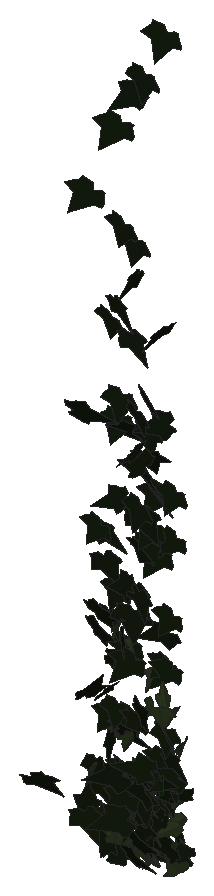
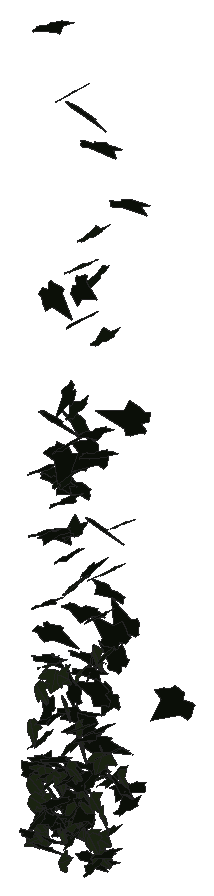
# SketchUp Ruby script. Lengths in inches.
U = 1.inch
M = Sketchup.active_model
def pt(a) = Geom::Point3d.new(a.map { |v| v * U })
def face(e, loops, mat)
  f = e.add_face(loops[0].map { |a| pt(a) })
  loops[1..].each { |l| e.add_face(l.map { |a| pt(a) }).erase! }
  f.material = f.back_material = mat if mat
  f
end
# faces: each face lists its corners as indices into pts; further lists are holes
def faces(e, pts, list, mat = nil) = list.each { |f| face(e, (f[0].is_a?(Array) ? f : [f]).map { |l| l.map { |i| pts[i] } }, mat) }
# xy, xz, yz: faces in a plane at the given z, y or x. An outline is a flat list of corners, or four numbers for a rectangle; further outlines are holes
def ring(l) = l.size == 4 ? [[l[0], l[1]], [l[2], l[1]], [l[2], l[3]], [l[0], l[3]]] : l.each_slice(2).to_a
def flat(e, list, mat, &to3) = list.each { |f| face(e, (f[0].is_a?(Array) ? f : [f]).map { |l| ring(l).map { |u, v| to3.(u, v) } }, mat) }
def xy(e, z, list, mat = nil) = flat(e, list, mat) { |x, y| [x, y, z] }
def xz(e, y, list, mat = nil) = flat(e, list, mat) { |x, z| [x, y, z] }
def yz(e, x, list, mat = nil) = flat(e, list, mat) { |y, z| [x, y, z] }
def lines(e, pts, list) = list.each { |a, b| e.add_line(pt(pts[a]), pt(pts[b])) }
# prism: a flat outline (further loops are holes) pulled along v
def prism(e, loops, v, mat = nil)
  f = face(e, loops, mat); d = Geom::Vector3d.new(v.map { |x| x * U })
  f.pushpull(f.normal.samedirection?(d) ? d.length : -d.length)
end
def box(e, o, s, mat = nil) = prism(e, [[o, [o[0] + s[0], o[1], o[2]], [o[0] + s[0], o[1] + s[1], o[2]], [o[0], o[1] + s[1], o[2]]]], [0, 0, s[2]], mat)
def at(x, y, z, deg = 0) = Geom::Transformation.translation(pt([x, y, z])) * Geom::Transformation.rotation(ORIGIN, Z_AXIS, deg.degrees)
def axes(o, x, y, z) = Geom::Transformation.new([*x, 0, *y, 0, *z, 0, *pt(o).to_a, 1])
def part(name) = M.definitions.add(name)
# library, detail: a bought-in or finely detailed component or shape, given as its bounding box
def library(name, o, s) = part(name).tap { |d| box(d.entities, o, s) }
def detail(e, o, s) = box(e.add_group.entities, o, s)
def put(e, d, t, mat = nil) = e.add_instance(d, t).tap { |i| i.material = mat if mat }
def group(e, t, mat = nil) = e.add_group.tap { |g| g.transformation = t; g.material = mat if mat }.entities
root = M.entities
M.materials.add("1026 AP 7946 SUNNY SIDE UP").color = [254, 231, 186]
M.materials.add("efeu1").color = [18, 25, 13]
M.materials.add("efeu2").color = [43, 57, 29]
c1 = part("ivyleaf_9")
p = [[1.54,2.16,1.25],[1.36,2.04,1.19],[-0.21,0.99,0.68],[-0.71,1.11,0.82],[-0.85,0.86,0.67],[-0.8,0.17,0.21],
  [-0.9,-0.01,0.1],[-0.67,-0.16,-0.02],[-0.08,-0.08,-0.05],[-0.03,-0.6,-0.4],[0.65,-0.88,-0.66],[0.83,-0.6,-0.49],
  [1.29,-0.42,-0.43],[1.8125,-0.07,-0.26],[1.21,0.44,0.15]]
faces(c1.entities,p,[[0,1,2,3,4,5,6,7,8,9,10,11,12,13,14]],"efeu1")
c2 = part("ivyleaf_10")
p = [[0,0.5,-0.03],[-0.0625,2.02,-0.43],[-0.19,2.01,-0.46],[-0.54,1.05,-0.29],[-0.52,0.625,-0.18],[-0.83,0.76,-0.28],
  [-1.16,0.64,-0.33],[-1.15,0.33,-0.24],[-0.77,-0.39,0.02],[-0.3,-0.51,0.16],[0.04,-0.48,0.23],[-0.02,2.01,-0.4375],
  [-0.06,2.01,-0.43],[0.04,-0.49,0.23],[0.67,-0.49,0.14],[1.38,0.36,-0.2],[1.375,0.51,-0.24],[0.81,0.65,-0.19],
  [0.62,0.59,-0.15],[0.6,1.09,-0.28],[0.5,1.23,-0.31]]
faces(c2.entities,p,[[0,1,2,3,4,5,6,7,8,9,10],[11,12,0,13,14,15,16,17,18,19,20]],"efeu2")
put(root,c1,axes([133.82,210.72,323.58],[-0.60668,-0.24823,0.06336],[-0.05107,-0.0654,-0.47148],[0.39941,-0.38542,0.03595]),"1026 AP 7946 SUNNY SIDE UP")
put(root,c1,axes([133.66,212.19,296.95],[-0.25305,-0.29819,0.20557],[-0.05268,-0.20708,-0.34492],[0.5632,-0.15335,0.0601]),"1026 AP 7946 SUNNY SIDE UP")
put(root,c1,axes([133.34,211.92,306.15],[0.33807,-0.31526,-0.18809],[0.02962,0.21944,-0.36986],[0.57067,0.17537,0.13063]),"1026 AP 7946 SUNNY SIDE UP")
put(root,c1,axes([133.68,211.13,295.07],[-0.4086,-0.0556,-0.27243],[0.42204,-0.01442,-0.26899],[0.04493,-0.37025,0.04917]),"1026 AP 7946 SUNNY SIDE UP")
put(root,c1,axes([133.33,211.56,301.29],[0.15223,-0.12655,0.42868],[0.33324,-0.35939,-0.16521],[0.59846,0.23231,-0.01705]),"1026 AP 7946 SUNNY SIDE UP")
put(root,c1,axes([133.55,212.28,301.875],[0.15265,-0.38546,0.07112],[0.00869,-0.07203,-0.40973],[0.6163,0.09649,-0.01184]),"1026 AP 7946 SUNNY SIDE UP")
put(root,c1,axes([133.79,212.14,292],[-0.25038,-0.34865,0.09324],[-0.02708,-0.09364,-0.39473],[0.56654,-0.15856,0.02234]),"1026 AP 7946 SUNNY SIDE UP")
put(root,c1,axes([133.27,210.27,312.67],[0.43109,-0.05163,0.40474],[0.59998,-0.09579,-0.28762],[0.16976,0.46965,-0.01128]),"1026 AP 7946 SUNNY SIDE UP")
put(root,c1,axes([133.99,210.24,293.31],[-0.29871,-0.18114,0.34824],[0.33996,0.26238,0.27073],[-0.4998,0.28673,-0.02398]),"1026 AP 7946 SUNNY SIDE UP")
put(root,c2,axes([133.96,210.66,295.04],[0.24035,-0.33847,0.14317],[0.06117,-0.13682,-0.38287],[0.57322,0.15652,-0.01917]),"1026 AP 7946 SUNNY SIDE UP")
put(root,c2,axes([133.95,212.01,296.65],[-0.40052,-0.26352,-0.09672],[0.1592,0.02939,-0.37375],[0.40921,-0.26936,0.05074]),"1026 AP 7946 SUNNY SIDE UP")
put(root,c2,axes([133.86,212.07,293.75],[0.28119,-0.23923,0.25103],[0.20504,-0.20803,-0.3085],[0.4979,0.22078,-0.01472]),"1026 AP 7946 SUNNY SIDE UP")
put(root,c1,axes([133.72,211.73,304.91],[-0.21133,-0.18347,-0.35122],[0.53318,0.11628,-0.20211],[0.29082,-0.34651,0.11532]),"1026 AP 7946 SUNNY SIDE UP")
put(root,c1,axes([133.61,211.36,302.28],[0.09541,-0.1357,0.44882],[0.50077,-0.30322,-0.14451],[0.51545,0.31971,0.05732]),"1026 AP 7946 SUNNY SIDE UP")
put(root,c1,axes([134.56,211.88,308.03],[-0.60402,0.14951,0.07455],[-0.13035,-0.01701,-0.42219],[-0.22565,-0.39037,0.04433]),"1026 AP 7946 SUNNY SIDE UP")
put(root,c1,axes([134.14,212.29,311.73],[-0.37368,-0.35693,0.00895],[0.01788,-0.02043,-0.44136],[0.56121,-0.23701,0.02002]),"1026 AP 7946 SUNNY SIDE UP")
put(root,c2,axes([134.28,212.02,301.69],[0.14177,-0.38008,0.04062],[0.00044,-0.04267,-0.40256],[0.60121,0.08966,-0.00929]),"1026 AP 7946 SUNNY SIDE UP")
put(root,c1,axes([134.2,212.32,312.8125],[-0.26833,-0.39268,0.00969],[0.01126,-0.0158,-0.44098],[0.61762,-0.17032,0.01225]),"1026 AP 7946 SUNNY SIDE UP")
put(root,c2,axes([134.41,211.54,291.43],[-0.29588,-0.2425,0.20288],[-0.04616,-0.21667,-0.30291],[0.49041,-0.1667,0.09389]),"1026 AP 7946 SUNNY SIDE UP")
put(root,c1,axes([133.82,212.08,299.85],[0.30048,-0.02764,-0.35985],[0.52008,0.14506,0.17552],[0.18113,-0.37065,0.09301]),"1026 AP 7946 SUNNY SIDE UP")
put(root,c1,axes([134.29,212.02,303.46],[-0.2156,-0.35734,0.18493],[-0.04474,-0.18271,-0.3937],[0.62864,-0.13556,0.0354]),"1026 AP 7946 SUNNY SIDE UP")
put(root,c2,axes([134.43,212.09,292.42],[0.03147,-0.36463,0.09676],[0.0125,-0.0957,-0.37675],[0.59275,0.02138,0.00281]),"1026 AP 7946 SUNNY SIDE UP")
put(root,c1,axes([134.23,211.52,296.3125],[-0.30033,0.02642,-0.41378],[0.58056,-0.16598,-0.19302],[-0.25267,-0.41277,0.04831]),"1026 AP 7946 SUNNY SIDE UP")
put(root,c1,axes([134.54,211.77,326.68],[-0.6333,-0.2444,-0.0129],[0.05878,-0.04029,-0.4824],[0.38018,-0.4009,0.0531]),"1026 AP 7946 SUNNY SIDE UP")
put(root,c1,axes([134.39,210.57,307.25],[-0.29378,-0.31279,0.22737],[-0.02894,-0.23985,-0.36472],[0.60286,-0.16394,0.09329]),"1026 AP 7946 SUNNY SIDE UP")
put(root,c1,axes([134.22,211.57,317.02],[-0.12608,-0.34417,0.27117],[0.10627,-0.27625,-0.34993],[0.67486,-0.0208,0.10576]),"1026 AP 7946 SUNNY SIDE UP")
put(root,c1,axes([134.52,210.65,298.96],[0.13676,0.33423,0.22093],[0.10528,0.20208,-0.3544],[-0.61386,0.10912,-0.01156]),"1026 AP 7946 SUNNY SIDE UP")
put(root,c1,axes([134.36,211.8,297.78],[-0.16284,-0.37763,0.07176],[-0.00004,-0.07436,-0.40334],[0.60443,-0.10174,0.01931]),"1026 AP 7946 SUNNY SIDE UP")
put(root,c1,axes([134.21,212.21,291.2],[0.14541,-0.33915,0.14103],[0.05987,-0.13351,-0.36292],[0.5731,0.1,0.00213]),"1026 AP 7946 SUNNY SIDE UP")
put(root,c1,axes([134.34,211.875,311.58],[0.59164,0.20341,0.06637],[0.11618,-0.00418,-0.43889],[-0.31416,0.38153,-0.03732]),"1026 AP 7946 SUNNY SIDE UP")
put(root,c2,axes([134.59,211.8,294.25],[0.02544,-0.3266,0.17951],[0.08652,-0.17221,-0.33524],[0.57699,0.04022,0.04236]),"1026 AP 7946 SUNNY SIDE UP")
put(root,c2,axes([134.64,211.96,292.51],[-0.05107,-0.30534,0.2054],[0.06856,-0.2037,-0.31254],[0.5708,-0.00285,0.05592]),"1026 AP 7946 SUNNY SIDE UP")
put(root,c1,axes([134.33,206.06,296.71],[0.68139,0.18295,0.08218],[0.1391,-0.0079,-0.48277],[-0.28059,0.44037,-0.03978]),"1026 AP 7946 SUNNY SIDE UP")
put(root,c1,axes([134.78,212.18,300.74],[-0.49426,-0.2598,0.00472],[0.02257,-0.02685,-0.41915],[0.408,-0.31325,0.0289]),"1026 AP 7946 SUNNY SIDE UP")
put(root,c1,axes([135.18,211.28,290.73],[-0.0689,0.10775,0.39434],[-0.58598,0.12157,-0.07862],[-0.21553,-0.36496,0.08768]),"1026 AP 7946 SUNNY SIDE UP")
put(root,c1,axes([134.82,211.55,301.38],[0.26557,-0.13416,-0.41163],[-0.53677,0.20753,-0.21965],[0.38678,0.38013,-0.02219]),"1026 AP 7946 SUNNY SIDE UP")
put(root,c1,axes([134.8125,212.13,297.38],[-0.26562,-0.33325,0.12495],[-0.05149,-0.12121,-0.3848],[0.55628,-0.17034,0.02404]),"1026 AP 7946 SUNNY SIDE UP")
put(root,c1,axes([134.5,210.21,294.77],[0.35404,-0.39938,-0.0663],[-0.00638,0.06883,-0.4709],[0.63549,0.22319,0.03221]),"1026 AP 7946 SUNNY SIDE UP")
put(root,c1,axes([134.91,211.58,294.9],[-0.28978,-0.25449,0.22169],[-0.03128,-0.2386,-0.30758],[0.52458,-0.15481,0.10412]),"1026 AP 7946 SUNNY SIDE UP")
put(root,c2,axes([134.91,210.8125,291.7],[0.05351,-0.24568,0.31772],[0.1384,-0.29844,-0.25552],[0.60612,0.08984,0.0303]),"1026 AP 7946 SUNNY SIDE UP")
put(root,c1,axes([135.31,212.09,328.36],[-0.73472,0.06447,-0.02271],[0.02615,-0.04287,-0.48441],[-0.1041,-0.46582,0.03864]),"1026 AP 7946 SUNNY SIDE UP")
put(root,c1,axes([134.76,209.11,293.73],[-0.11412,-0.34985,-0.26262],[0.09045,0.24636,-0.3666],[0.67276,-0.09246,0.00474]),"1026 AP 7946 SUNNY SIDE UP")
put(root,c1,axes([134.86,210.5,291.83],[-0.1567,-0.28965,0.25415],[0.00849,-0.25772,-0.30894],[0.59988,-0.07202,0.07076]),"1026 AP 7946 SUNNY SIDE UP")
put(root,c2,axes([134.9,212.39,300.5625],[-0.19719,-0.12594,0.37004],[0.27359,-0.35603,-0.06797],[0.53351,0.13603,0.17162]),"1026 AP 7946 SUNNY SIDE UP")
put(root,c1,axes([134.91,212.4,320.7],[-0.18624,-0.3989,0.16842],[0.06274,-0.18124,-0.42103],[0.67633,-0.09303,0.08543]),"1026 AP 7946 SUNNY SIDE UP")
put(root,c1,axes([134.75,211.5625,295.08],[0.26777,-0.31096,0.16305],[0.0778,-0.15479,-0.36499],[0.54438,0.17508,-0.02804]),"1026 AP 7946 SUNNY SIDE UP")
put(root,c1,axes([135.0625,211.61,293.51],[0.16703,0.26443,0.28928],[0.17846,0.2553,-0.29198],[-0.57784,0.15529,-0.00656]),"1026 AP 7946 SUNNY SIDE UP")
put(root,c1,axes([134.93,211.55,321.9],[-0.18521,-0.37083,0.26398],[0.05198,-0.27333,-0.39026],[0.70875,-0.07686,0.09761]),"1026 AP 7946 SUNNY SIDE UP")
put(root,c2,axes([135.21,211.87,296.83],[0.28673,-0.34688,-0.06128],[-0.03008,0.05491,-0.4033],[0.55206,0.18315,0.00985]),"1026 AP 7946 SUNNY SIDE UP")
put(root,c2,axes([135.33,211.98,293.67],[-0.3898,-0.29559,0.02535],[0.00657,-0.03772,-0.39664],[0.46657,-0.24642,0.02676]),"1026 AP 7946 SUNNY SIDE UP")
put(root,c1,axes([135.42,211.84,319.41],[-0.20913,0.11837,-0.43304],[0.3483,-0.3612,-0.17882],[-0.59294,-0.25392,0.04769]),"1026 AP 7946 SUNNY SIDE UP")
put(root,c1,axes([135.18,211.89,292.63],[0.12533,-0.36042,0.0502],[0.00201,-0.0517,-0.38044],[0.57232,0.07911,-0.00966]),"1026 AP 7946 SUNNY SIDE UP")
put(root,c1,axes([135.49,211.84,297.39],[-0.30432,-0.2498,0.22047],[-0.01702,-0.24483,-0.30391],[0.5184,-0.15468,0.11945]),"1026 AP 7946 SUNNY SIDE UP")
put(root,c1,axes([135.74,211.18,300.74],[-0.66388,-0.12672,-0.03313],[0.06712,-0.03342,-0.45203],[0.19402,-0.42205,0.04303]),"1026 AP 7946 SUNNY SIDE UP")
put(root,c1,axes([135.42,212.375,329.1],[-0.14341,-0.43391,0.17612],[0.02215,-0.17917,-0.45524],[0.73443,-0.07932,0.04812]),"1026 AP 7946 SUNNY SIDE UP")
put(root,c2,axes([135.97,210.77,291.8],[-0.17644,0.18244,0.33796],[-0.48992,0.14388,-0.19199],[-0.32661,-0.31437,0.10542]),"1026 AP 7946 SUNNY SIDE UP")
put(root,c1,axes([135.33,212.19,293.625],[0.33164,-0.32568,0.00831],[-0.01525,-0.01808,-0.3994],[0.5121,0.21037,-0.01727]),"1026 AP 7946 SUNNY SIDE UP")
put(root,c2,axes([135.98,211.58,295.16],[-0.03157,-0.01101,-0.4141],[-0.39045,0.31681,0.00569],[0.49719,0.2481,-0.02183]),"1026 AP 7946 SUNNY SIDE UP")
put(root,c1,axes([135.8,210.85,304.53],[-0.18813,-0.07411,0.42061],[-0.33519,-0.35408,-0.1325],[0.56055,-0.2366,0.06193]),"1026 AP 7946 SUNNY SIDE UP")
put(root,c1,axes([136.07,209.86,295.71],[-0.07957,-0.11254,-0.42497],[-0.28797,-0.36895,0.12487],[-0.60648,0.18995,-0.00353]),"1026 AP 7946 SUNNY SIDE UP")
put(root,c1,axes([135.28,210.98,297.2],[0.54552,-0.03117,0.16177],[0.23588,-0.06875,-0.35551],[0.08868,0.37463,-0.0495]),"1026 AP 7946 SUNNY SIDE UP")
put(root,c2,axes([135.82,210.98,297.14],[-0.12423,-0.37052,0.11899],[-0.01772,-0.11778,-0.39075],[0.611,-0.07875,0.01286]),"1026 AP 7946 SUNNY SIDE UP")
put(root,c1,axes([135.46,212.09,292.125],[0.25475,-0.33988,0.07992],[0.03048,-0.07876,-0.388],[0.54802,0.16238,-0.01557]),"1026 AP 7946 SUNNY SIDE UP")
put(root,c1,axes([135.65,212.23,306.15],[-0.06607,-0.4114,0.04659],[-0.00283,-0.04762,-0.42629],[0.65119,-0.04195,0.00288]),"1026 AP 7946 SUNNY SIDE UP")
put(root,c1,axes([135.71,211.24,303.09],[-0.45418,-0.29081,-0.20915],[0.26634,0.11452,-0.42],[0.48828,-0.33297,0.03455]),"1026 AP 7946 SUNNY SIDE UP")
put(root,c1,axes([135.66,212.3,311.63],[-0.02585,-0.42879,0.03411],[0.00054,-0.03559,-0.44226],[0.67654,-0.01636,0.00166]),"1026 AP 7946 SUNNY SIDE UP")
put(root,c1,axes([135.48,211.42,294.59],[0.61392,0.00895,-0.10197],[0.1466,0.10659,0.3892],[0.05437,-0.38844,0.102]),"1026 AP 7946 SUNNY SIDE UP")
put(root,c2,axes([135.92,211.04,293.55],[0.00561,-0.37974,-0.0911],[0.03371,0.08634,-0.39008],[0.6114,-0.00127,0.02234]),"1026 AP 7946 SUNNY SIDE UP")
put(root,c1,axes([135.7,208.01,300.45],[0.40012,0.37029,0.18091],[-0.19248,-0.126,0.46125],[0.61351,-0.28103,0.02673]),"1026 AP 7946 SUNNY SIDE UP")
put(root,c1,axes([135.64,210.0625,319.01],[0.33537,-0.39827,-0.01628],[-0.02542,0.0067,-0.46525],[0.62609,0.21361,-0.01017]),"1026 AP 7946 SUNNY SIDE UP")
put(root,c1,axes([135.93,211.69,310.79],[0.56732,0.27477,-0.09247],[-0.08152,-0.08224,-0.46642],[-0.44793,0.36297,-0.03223]),"1026 AP 7946 SUNNY SIDE UP")
put(root,c1,axes([136.26,210.14,294.65],[-0.64164,-0.13278,0.02054],[-0.01125,-0.04458,-0.44041],[0.21101,-0.40615,0.03896]),"1026 AP 7946 SUNNY SIDE UP")
put(root,c1,axes([135.74,211.45,312.93],[0.08527,-0.35595,0.25847],[0.09956,-0.24575,-0.37174],[0.67933,0.0807,0.02204]),"1026 AP 7946 SUNNY SIDE UP")
put(root,c1,axes([135.78,211.4,304.28],[0.19016,-0.43155,0.02402],[-0.00741,-0.02807,-0.46171],[0.67974,0.12042,-0.01175]),"1026 AP 7946 SUNNY SIDE UP")
put(root,c1,axes([135.99,211.57,313.84],[0.52321,-0.18581,-0.26989],[-0.3602,0.12494,-0.39188],[0.35206,0.40397,0.00015]),"1026 AP 7946 SUNNY SIDE UP")
put(root,c2,axes([136.22,211.76,298.47],[0.29525,-0.31992,-0.1046],[-0.08029,0.08565,-0.38165],[0.52075,0.19459,0.00046]),"1026 AP 7946 SUNNY SIDE UP")
put(root,c2,axes([136.07,212.07,290.74],[0.03324,-0.07815,0.3665],[0.17392,-0.33862,-0.08528],[0.5464,0.11254,0.00485]),"1026 AP 7946 SUNNY SIDE UP")
put(root,c1,axes([136.02,211.7,294.7],[-0.10511,-0.37939,0.07883],[-0.01153,-0.07858,-0.39728],[0.60914,-0.06695,0.00608]),"1026 AP 7946 SUNNY SIDE UP")
put(root,c1,axes([136,212.1,292.94],[-0.00788,-0.3421,0.1335],[-0.00636,-0.13149,-0.35323],[0.57628,-0.00613,-0.00207]),"1026 AP 7946 SUNNY SIDE UP")
put(root,c1,axes([135.82,211.875,309.83],[0.32299,-0.36854,0.11682],[0.05244,-0.11339,-0.43455],[0.60502,0.20658,-0.0247]),"1026 AP 7946 SUNNY SIDE UP")
put(root,c2,axes([136.0625,211.93,291.82],[-0.00393,-0.24303,-0.28876],[0.14968,-0.26995,0.23986],[-0.56211,-0.07018,0.06589]),"1026 AP 7946 SUNNY SIDE UP")
put(root,c1,axes([136,211.28,304.15],[0.08128,-0.43445,0.10261],[-0.00393,-0.10304,-0.45108],[0.70171,0.04974,-0.01441]),"1026 AP 7946 SUNNY SIDE UP")
put(root,c1,axes([135.95,210.74,317.12],[0.14349,-0.42604,-0.11053],[0.05474,0.11381,-0.44443],[0.68772,0.07983,0.05843]),"1026 AP 7946 SUNNY SIDE UP")
put(root,c2,axes([136.22,211.97,299.87],[-0.03563,-0.22603,0.34071],[0.2075,-0.31827,-0.2158],[0.59649,0.09721,0.09542]),"1026 AP 7946 SUNNY SIDE UP")
put(root,c1,axes([136.62,210.47,311.78],[-0.43154,0.30728,-0.15362],[0.11082,-0.1385,-0.4235],[-0.52673,-0.28089,0.03676]),"1026 AP 7946 SUNNY SIDE UP")
put(root,c1,axes([135.95,211.68,293.51],[0.40393,-0.24209,0.1592],[0.14265,-0.13025,-0.36311],[0.42971,0.2708,-0.02911]),"1026 AP 7946 SUNNY SIDE UP")
put(root,c1,axes([136.87,212.18,302.07],[-0.00947,-0.01534,-0.41127],[-0.41586,-0.29898,0.0142],[-0.47065,0.26448,-0.00428]),"1026 AP 7946 SUNNY SIDE UP")
put(root,c1,axes([136.5625,212.24,295.75],[-0.40658,-0.25142,0.12086],[-0.04806,-0.13546,-0.36486],[0.43456,-0.25021,0.07272]),"1026 AP 7946 SUNNY SIDE UP")
put(root,c1,axes([136.33,211.1,306.46],[-0.19397,-0.248,0.34409],[0.11422,-0.3572,-0.24665],[0.64589,-0.01131,0.14695]),"1026 AP 7946 SUNNY SIDE UP")
put(root,c1,axes([136.25,211.94,292.25],[0.08817,-0.26205,0.26743],[0.10218,-0.25298,-0.27744],[0.5726,0.0855,0.00833]),"1026 AP 7946 SUNNY SIDE UP")
put(root,c1,axes([136.99,211.99,312.5],[-0.64603,0.11896,0.11372],[-0.1837,-0.01088,-0.43862],[-0.17608,-0.42511,0.04037]),"1026 AP 7946 SUNNY SIDE UP")
put(root,c1,axes([136.29,210.95,298.27],[-0.09622,0.07132,0.47583],[0.14783,-0.45401,0.08247],[0.71921,0.10286,0.04671]),"1026 AP 7946 SUNNY SIDE UP")
put(root,c1,axes([136.36,210.96,294.38],[-0.41585,-0.14136,-0.3441],[0.5131,0.08546,-0.30366],[0.24628,-0.41674,0.05163]),"1026 AP 7946 SUNNY SIDE UP")
put(root,c1,axes([137.07,211.82,292.19],[-0.48813,0.08511,0.22509],[-0.34523,0.01951,-0.3298],[-0.12745,-0.37884,0.03126]),"1026 AP 7946 SUNNY SIDE UP")
put(root,c2,axes([136.66,211.66,294.6],[0.02273,-0.38106,0.03308],[-0.00087,-0.03431,-0.39304],[0.60159,0.01435,-0.00182]),"1026 AP 7946 SUNNY SIDE UP")
put(root,c1,axes([136.4375,212.04,293.66],[-0.05615,-0.33851,-0.14538],[0.06033,0.13562,-0.34912],[0.57234,-0.0475,0.02254]),"1026 AP 7946 SUNNY SIDE UP")
put(root,c1,axes([136.6875,212.35,300.37],[-0.3643,-0.2469,0.22384],[-0.04065,-0.25283,-0.32376],[0.51701,-0.19385,0.13227]),"1026 AP 7946 SUNNY SIDE UP")
put(root,c1,axes([136.16,210.33,291.67],[0.33586,-0.19045,0.32991],[0.35126,-0.23152,-0.2957],[0.47071,0.30866,-0.01474]),"1026 AP 7946 SUNNY SIDE UP")
put(root,c1,axes([136.52,212.04,292.83],[-0.30053,-0.07554,-0.31622],[0.48887,0.01714,-0.20397],[0.08614,-0.36083,0.0543]),"1026 AP 7946 SUNNY SIDE UP")
put(root,c1,axes([136.48,211.05,292.64],[-0.28614,-0.06051,-0.35241],[0.54179,0.01465,-0.19161],[0.06527,-0.38689,0.04554]),"1026 AP 7946 SUNNY SIDE UP")
put(root,c1,axes([137.25,210.02,311.41],[-0.35065,0.36541,0.20313],[-0.25482,0.12695,-0.43504],[-0.59942,-0.26772,0.06612]),"1026 AP 7946 SUNNY SIDE UP")
put(root,c1,axes([136.9,211.68,309.3],[-0.60177,-0.16894,-0.06389],[0.10664,-0.00281,-0.4299],[0.26155,-0.38754,0.02827]),"1026 AP 7946 SUNNY SIDE UP")
put(root,c1,axes([136.59,211.92,306.83],[-0.03139,-0.39617,-0.14437],[0.05481,0.136,-0.40695],[0.65732,-0.03026,0.02704]),"1026 AP 7946 SUNNY SIDE UP")
put(root,c2,axes([136.6,210.74,291.84],[-0.49745,-0.07838,-0.24301],[0.37231,0.01882,-0.3341],[0.11677,-0.39391,0.02999]),"1026 AP 7946 SUNNY SIDE UP")
put(root,c1,axes([136.74,210.42,309.07],[-0.14972,-0.40445,0.20648],[-0.04879,-0.20084,-0.42898],[0.7097,-0.09913,0.01407]),"1026 AP 7946 SUNNY SIDE UP")
put(root,c1,axes([136.74,212.04,294.92],[-0.11205,-0.38669,-0.01742],[0.01121,0.01364,-0.40497],[0.60838,-0.07147,0.00425]),"1026 AP 7946 SUNNY SIDE UP")
put(root,c1,axes([137.33,212.22,291.22],[-0.56022,0.07019,0.16726],[-0.27567,-0.09836,-0.35399],[-0.03222,-0.37881,0.12046]),"1026 AP 7946 SUNNY SIDE UP")
put(root,c1,axes([136.87,212.03,331.85],[-0.35472,-0.41895,0.0602],[-0.01694,-0.0632,-0.49012],[0.66545,-0.22493,0.01961]),"1026 AP 7946 SUNNY SIDE UP")
put(root,c1,axes([136.93,211.07,307.87],[-0.29227,-0.3641,0.17411],[-0.08194,-0.16508,-0.42123],[0.62723,-0.19122,0.02611]),"1026 AP 7946 SUNNY SIDE UP")
put(root,c1,axes([136.51,211.47,309.46],[0.38086,-0.34229,0.2021],[0.13985,-0.17923,-0.43207],[0.60595,0.25651,-0.02731]),"1026 AP 7946 SUNNY SIDE UP")
put(root,c1,axes([137.0625,211.4,306.38],[-0.49657,-0.27766,0.02059],[0.00617,-0.03703,-0.43229],[0.43787,-0.31437,0.02943]),"1026 AP 7946 SUNNY SIDE UP")
put(root,c1,axes([136.65,210.55,308.66],[-0.28623,-0.16312,-0.40021],[0.5141,0.21065,-0.24831],[0.41575,-0.37278,0.03151]),"1026 AP 7946 SUNNY SIDE UP")
put(root,c1,axes([137.2,211.99,300.46],[-0.5299,-0.19283,0.0467],[-0.0398,-0.04898,-0.39911],[0.30933,-0.33664,0.02866]),"1026 AP 7946 SUNNY SIDE UP")
put(root,c1,axes([136.73,211.97,292.9],[0.53986,-0.17904,-0.00943],[-0.03656,-0.02706,-0.39745],[0.27943,0.34236,-0.03378]),"1026 AP 7946 SUNNY SIDE UP")
put(root,c1,axes([137.45,208.46,294.61],[-0.58091,-0.14113,0.27254],[-0.35898,-0.14169,-0.40592],[0.30735,-0.43223,0.041]),"1026 AP 7946 SUNNY SIDE UP")
put(root,c2,axes([136.94,212.13,295.05],[0.57468,0.10061,0.01599],[0.03723,-0.02993,-0.38901],[-0.15555,0.36456,-0.03405]),"1026 AP 7946 SUNNY SIDE UP")
put(root,c1,axes([136.54,210.22,292.5],[0.19809,-0.16534,0.40847],[0.42424,-0.29234,-0.2151],[0.5274,0.29726,0.01961]),"1026 AP 7946 SUNNY SIDE UP")
put(root,c1,axes([136.85,211.99,294.29],[0.14117,-0.35932,0.04259],[0.00293,-0.04424,-0.3817],[0.56909,0.08936,-0.0086]),"1026 AP 7946 SUNNY SIDE UP")
put(root,c1,axes([137.15,212.34,306.77],[-0.36755,-0.29535,0.16572],[-0.05496,-0.17549,-0.38132],[0.52724,-0.22419,0.07578]),"1026 AP 7946 SUNNY SIDE UP")
put(root,c1,axes([137.23,211.36,293.43],[-0.51408,0.09661,-0.23797],[0.32108,-0.11853,-0.34866],[-0.22921,-0.38269,0.04532]),"1026 AP 7946 SUNNY SIDE UP")
put(root,c1,axes([137.66,209.81,296.5],[-0.3388,-0.00565,0.38109],[-0.55633,-0.1221,-0.21492],[0.1702,-0.41034,0.05609]),"1026 AP 7946 SUNNY SIDE UP")
put(root,c1,axes([137.07,211.83,297.41],[-0.1236,-0.38822,0.0253],[0.00169,-0.02752,-0.40816],[0.61188,-0.07834,0.00623]),"1026 AP 7946 SUNNY SIDE UP")
put(root,c1,axes([137.21,212.01,303.09],[-0.28582,-0.32484,0.17359],[-0.06096,-0.17204,-0.38159],[0.57352,-0.18018,0.04595]),"1026 AP 7946 SUNNY SIDE UP")
put(root,c1,axes([137.18,210.12,295.14],[0.29822,-0.38912,-0.1865],[0.15335,-0.15119,0.44459],[-0.65567,-0.21234,0.01916]),"1026 AP 7946 SUNNY SIDE UP")
put(root,c1,axes([137.76,211.21,292.2],[0.01559,0.0209,-0.44575],[-0.66827,-0.08392,-0.0147],[-0.13282,0.42471,0.02162]),"1026 AP 7946 SUNNY SIDE UP")
put(root,c1,axes([137.62,211.82,295.23],[-0.52377,-0.13052,0.12954],[-0.16609,-0.07589,-0.36768],[0.23257,-0.34813,0.02917]),"1026 AP 7946 SUNNY SIDE UP")
put(root,c1,axes([137.23,212.35,292.4],[-0.00623,-0.23969,0.28554],[0.03286,-0.27824,-0.24799],[0.57687,0.01326,0.01721]),"1026 AP 7946 SUNNY SIDE UP")
put(root,c1,axes([137.24,212.04,295.05],[0.00529,-0.36689,0.07101],[0.01007,-0.07094,-0.37835],[0.58752,0.00452,0.00585]),"1026 AP 7946 SUNNY SIDE UP")
put(root,c1,axes([137.68,210.94,317.95],[-0.26858,0.32238,-0.31819],[0.15897,-0.29617,-0.37558],[-0.68582,-0.1949,0.03755]),"1026 AP 7946 SUNNY SIDE UP")
put(root,c2,axes([137.5,210.875,298.99],[-0.54411,-0.17503,-0.03665],[0.06921,-0.01063,-0.39842],[0.27186,-0.3476,0.02808]),"1026 AP 7946 SUNNY SIDE UP")
put(root,c2,axes([137.48,211.95,291.85],[0.12928,-0.29463,0.21824],[0.05742,-0.21111,-0.31583],[0.56925,0.08821,-0.01771]),"1026 AP 7946 SUNNY SIDE UP")
put(root,c2,axes([137.28,211.88,291.47],[-0.07354,-0.1493,-0.34462],[0.36298,0.24877,-0.14655],[0.44569,-0.22724,0.06249]),"1026 AP 7946 SUNNY SIDE UP")
put(root,c2,axes([137.77,211.57,292.99],[-0.19918,-0.15562,0.32264],[-0.20307,-0.28973,-0.20325],[0.51237,-0.17533,0.04487]),"1026 AP 7946 SUNNY SIDE UP")
put(root,c2,axes([137.62,211.75,298.65],[0.04282,-0.36749,0.12153],[-0.00415,-0.12053,-0.38016],[0.60789,0.02506,-0.01116]),"1026 AP 7946 SUNNY SIDE UP")
put(root,c1,axes([138.04,212.01,291.4],[-0.40591,0.07395,0.2766],[-0.43418,-0.0248,-0.26702],[-0.05184,-0.37133,0.07065]),"1026 AP 7946 SUNNY SIDE UP")
put(root,c2,axes([137.66,212.13,294.22],[-0.04788,-0.33748,0.20151],[-0.01709,-0.19731,-0.35018],[0.61462,-0.03177,0.00596]),"1026 AP 7946 SUNNY SIDE UP")
put(root,c2,axes([137.66,210.95,299.46],[0.00313,0.36355,-0.14408],[-0.02206,0.1419,0.37509],[0.61326,0.00325,0.01423]),"1026 AP 7946 SUNNY SIDE UP")
put(root,c1,axes([137.72,211.76,294.34],[0.35371,0.09048,0.34188],[-0.51204,-0.06978,0.24698],[0.17176,-0.39436,0.03223]),"1026 AP 7946 SUNNY SIDE UP")
put(root,c1,axes([137.33,211.7,296.3],[0.29262,-0.32049,-0.08787],[-0.03106,0.08484,-0.38043],[0.51982,0.18548,0.02673]),"1026 AP 7946 SUNNY SIDE UP")
put(root,c1,axes([137.26,211.45,297.54],[0.33053,-0.15578,-0.35547],[0.52082,-0.11342,0.26063],[-0.28568,-0.38701,0.06388]),"1026 AP 7946 SUNNY SIDE UP")
put(root,c2,axes([137.74,211.96,293.22],[-0.09804,-0.23539,0.29296],[-0.00762,-0.28919,-0.24824],[0.58203,-0.04344,0.0461]),"1026 AP 7946 SUNNY SIDE UP")
put(root,c1,axes([137.625,211.71,309.47],[-0.26222,-0.35073,0.1519],[-0.0292,-0.15545,-0.3981],[0.59875,-0.16118,0.04711]),"1026 AP 7946 SUNNY SIDE UP")
put(root,c2,axes([137.78,212.0625,296.93],[0.00781,-0.38885,-0.0839],[-0.01831,0.07906,-0.40002],[0.62372,0.00719,-0.0107]),"1026 AP 7946 SUNNY SIDE UP")
put(root,c2,axes([137.9,211.59,290.91],[-0.29745,-0.25165,-0.24453],[-0.23582,-0.18232,0.32315],[-0.48846,0.24127,-0.0071]),"1026 AP 7946 SUNNY SIDE UP")
